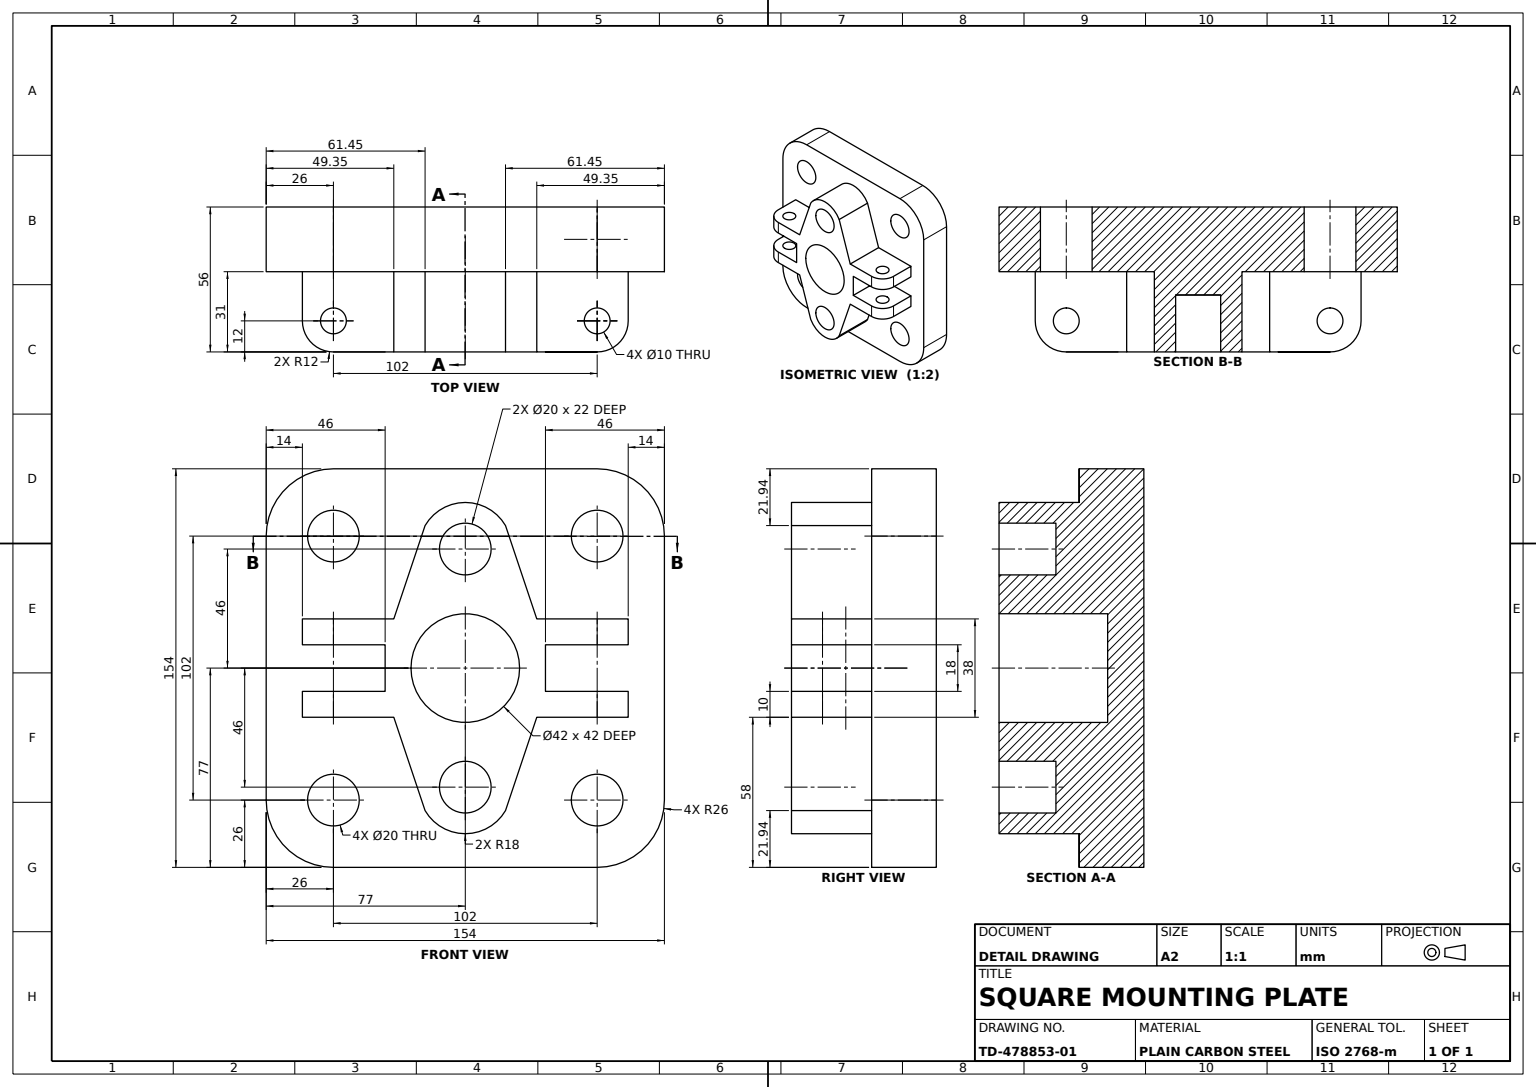
solid
v1 (26,-68,49)
v2 (26,-68,39)
e1 v1 v2 CIRCLE(AX(P(26,-68,44),D(0,-1,0),D(0,0,-1)),5)
v3 (26,-58,39)
e2 v3 v2 LINE
v4 (26,-58,49)
e3 v3 v4 CIRCLE(AX(P(26,-58,44),D(0,1,0),D(0,0,1)),5)
e4 v4 v1 LINE
face CYL(AX(P(26,-46,44),D(0,-1,0),D(0,0,-1)),5) rev [e1 -e2 e3 e4]
e5 v2 v1 CIRCLE(AX(P(26,-68,44),D(0,-1,0),D(0,0,-1)),5)
v5 (46,-68,56)
v6 (46,-68,25)
e6 v5 v6 LINE
v7 (26,-68,56)
e7 v5 v7 LINE
v8 (14,-68,44)
e8 v8 v7 CIRCLE(AX(P(26,-68,44),D(0,1,0),D(0,0,-1)),12)
v9 (14,-68,25)
e9 v8 v9 LINE
e10 v6 v9 LINE
face PLANE(AX(P(0,-68,56),D(0,-1,0),D(0,0,-1))) [-e5 -e1] [-e6 e7 -e8 e9 -e10]
v10 (128,-154,25)
v11 (128,-154,0)
e11 v10 v11 LINE
v12 (154,-128,0)
e12 v11 v12 CIRCLE(AX(P(128,-128,0),D(0,0,1),D(1,0,0)),26)
v13 (154,-128,25)
e13 v13 v12 LINE
e14 v10 v13 CIRCLE(AX(P(128,-128,25),D(0,0,1),D(1,0,0)),26)
face CYL(AX(P(128,-128,25),D(0,0,-1),D(-1,0,0)),26) [e11 e12 -e13 -e14]
v14 (154,-26,0)
e15 v12 v14 LINE
v15 (154,-26,25)
e16 v15 v14 LINE
e17 v13 v15 LINE
face PLANE(AX(P(154,-128,25),D(-1,0,0),D(0,0,1))) rev [e13 e15 -e16 -e17]
v16 (56,-77,14)
v17 (98,-77,14)
e18 v16 v17 CIRCLE(AX(P(77,-77,14),D(0,0,1),D(1,0,0)),21)
e19 v17 v16 CIRCLE(AX(P(77,-77,14),D(0,0,1),D(1,0,0)),21)
face PLANE(AX(P(77,-77,14),D(0,0,1),D(1,0,0))) [e18 e19]
v18 (36,-128,0)
v19 (16,-128,0)
e20 v18 v19 CIRCLE(AX(P(26,-128,0),D(0,0,1),D(1,0,0)),10)
v20 (36,-128,25)
e21 v18 v20 LINE
v21 (16,-128,25)
e22 v20 v21 CIRCLE(AX(P(26,-128,25),D(0,0,1),D(1,0,0)),10)
e23 v19 v21 LINE
face CYL(AX(P(26,-128,-17),D(0,0,1),D(1,0,0)),10) rev [-e20 e21 e22 -e23]
e24 v4 v3 CIRCLE(AX(P(26,-58,44),D(0,1,0),D(0,0,1)),5)
face CYL(AX(P(26,-46,44),D(0,-1,0),D(0,0,-1)),5) rev [e5 -e4 e24 e2]
v22 (67,-31,56)
v23 (87,-31,56)
e25 v22 v23 CIRCLE(AX(P(77,-31,56),D(0,0,1),D(1,0,0)),10)
e26 v23 v22 CIRCLE(AX(P(77,-31,56),D(0,0,1),D(1,0,0)),10)
v24 (87,-123,56)
v25 (67,-123,56)
e27 v24 v25 CIRCLE(AX(P(77,-123,56),D(0,0,1),D(1,0,0)),10)
e28 v25 v24 CIRCLE(AX(P(77,-123,56),D(0,0,1),D(1,0,0)),10)
v26 (92.552734,-21.938408,56)
v27 (61.447266,-21.938408,56)
e29 v26 v27 CIRCLE(AX(P(77,-31,56),D(0,0,1),D(1,0,0)),18)
v28 (49.353611,-58,56)
e30 v28 v27 LINE
v29 (26,-58,56)
e31 v29 v28 LINE
e32 v29 v7 LINE
v30 (46,-86,56)
e33 v30 v5 LINE
v31 (26,-86,56)
e34 v30 v31 LINE
v32 (26,-96,56)
e35 v31 v32 LINE
v33 (49.353611,-96,56)
e36 v32 v33 LINE
v34 (61.447266,-132.061592,56)
e37 v33 v34 LINE
v35 (92.552734,-132.061592,56)
e38 v34 v35 CIRCLE(AX(P(77,-123,56),D(0,0,1),D(1,0,0)),18)
v36 (104.646389,-96,56)
e39 v36 v35 LINE
v37 (128,-96,56)
e40 v37 v36 LINE
v38 (128,-86,56)
e41 v37 v38 LINE
v39 (108,-86,56)
e42 v39 v38 LINE
v40 (108,-68,56)
e43 v39 v40 LINE
v41 (128,-68,56)
e44 v40 v41 LINE
v42 (128,-58,56)
e45 v41 v42 LINE
v43 (104.646389,-58,56)
e46 v42 v43 LINE
e47 v43 v26 LINE
v44 (98,-77,56)
v45 (56,-77,56)
e48 v44 v45 CIRCLE(AX(P(77,-77,56),D(0,0,1),D(1,0,0)),21)
e49 v45 v44 CIRCLE(AX(P(77,-77,56),D(0,0,1),D(1,0,0)),21)
face PLANE(AX(P(0,0,56),D(0,0,1),D(1,0,0))) [-e25 -e26] [-e27 -e28] [e29 -e30 -e31 e32 -e7 -e33 e34 e35 e36 e37 e38 -e39 -e40 e41 -e42 e43 e44 e45 e46 e47] [-e48 -e49]
v46 (140,-96,44)
e50 v37 v46 CIRCLE(AX(P(128,-96,44),D(0,1,0),D(0,0,-1)),12)
v47 (140,-86,44)
e51 v47 v46 LINE
e52 v47 v38 CIRCLE(AX(P(128,-86,44),D(0,-1,0),D(0,0,1)),12)
face CYL(AX(P(128,-46,44),D(0,-1,0),D(0,0,-1)),12) [-e41 e50 -e51 e52]
v48 (26,-86,49)
v49 (26,-86,39)
e53 v48 v49 CIRCLE(AX(P(26,-86,44),D(0,-1,0),D(0,0,-1)),5)
e54 v49 v48 CIRCLE(AX(P(26,-86,44),D(0,-1,0),D(0,0,-1)),5)
v50 (46,-86,25)
v51 (14,-86,25)
e55 v50 v51 LINE
v52 (14,-86,44)
e56 v52 v51 LINE
e57 v52 v31 CIRCLE(AX(P(26,-86,44),D(0,1,0),D(0,0,-1)),12)
e58 v30 v50 LINE
face PLANE(AX(P(0,-86,56),D(0,-1,0),D(0,0,-1))) rev [e53 e54] [e55 -e56 e57 -e34 e58]
v53 (128,-86,49)
v54 (128,-86,39)
e59 v53 v54 CIRCLE(AX(P(128,-86,44),D(0,1,0),D(0,0,1)),5)
e60 v54 v53 CIRCLE(AX(P(128,-86,44),D(0,1,0),D(0,0,1)),5)
v55 (140,-86,25)
e61 v47 v55 LINE
v56 (108,-86,25)
e62 v56 v55 LINE
e63 v39 v56 LINE
face PLANE(AX(P(0,-86,56),D(0,1,0),D(0,0,1))) [-e59 -e60] [-e52 e61 -e62 -e63 e42]
v57 (14,-96,44)
v58 (14,-96,25)
e64 v57 v58 LINE
e65 v52 v57 LINE
e66 v51 v58 LINE
face PLANE(AX(P(14,0,56),D(1,0,0),D(0,0,-1))) rev [-e64 -e65 e56 e66]
v59 (138,-128,25)
v60 (118,-128,25)
e67 v59 v60 CIRCLE(AX(P(128,-128,25),D(0,0,1),D(1,0,0)),10)
v61 (118,-128,0)
e68 v61 v60 LINE
v62 (138,-128,0)
e69 v62 v61 CIRCLE(AX(P(128,-128,0),D(0,0,1),D(1,0,0)),10)
e70 v62 v59 LINE
face CYL(AX(P(128,-128,-17),D(0,0,1),D(1,0,0)),10) rev [e67 -e68 -e69 e70]
e71 v61 v62 CIRCLE(AX(P(128,-128,0),D(0,0,1),D(1,0,0)),10)
v63 (16,-26,0)
v64 (36,-26,0)
e72 v63 v64 CIRCLE(AX(P(26,-26,0),D(0,0,1),D(1,0,0)),10)
e73 v64 v63 CIRCLE(AX(P(26,-26,0),D(0,0,1),D(1,0,0)),10)
v65 (118,-26,0)
v66 (138,-26,0)
e74 v65 v66 CIRCLE(AX(P(128,-26,0),D(0,0,1),D(1,0,0)),10)
e75 v66 v65 CIRCLE(AX(P(128,-26,0),D(0,0,1),D(1,0,0)),10)
v67 (26,-154,0)
e76 v67 v11 LINE
v68 (0,-128,0)
e77 v68 v67 CIRCLE(AX(P(26,-128,0),D(0,0,1),D(1,0,0)),26)
v69 (0,-26,0)
e78 v69 v68 LINE
v70 (26,0,0)
e79 v70 v69 CIRCLE(AX(P(26,-26,0),D(0,0,1),D(1,0,0)),26)
v71 (128,0,0)
e80 v71 v70 LINE
e81 v14 v71 CIRCLE(AX(P(128,-26,0),D(0,0,1),D(-1,0,0)),26)
e82 v19 v18 CIRCLE(AX(P(26,-128,0),D(0,0,1),D(1,0,0)),10)
face PLANE(AX(P(26,-128,0),D(0,0,1),D(1,0,0))) rev [e71 e69] [e72 e73] [e74 e75] [-e15 -e12 -e76 -e77 -e78 -e79 -e80 -e81] [e82 e20]
v72 (128,-58,39)
v73 (128,-58,49)
e83 v72 v73 CIRCLE(AX(P(128,-58,44),D(0,-1,0),D(0,0,-1)),5)
v74 (128,-68,39)
e84 v72 v74 LINE
v75 (128,-68,49)
e85 v75 v74 CIRCLE(AX(P(128,-68,44),D(0,1,0),D(0,0,1)),5)
e86 v73 v75 LINE
face CYL(AX(P(128,-46,44),D(0,-1,0),D(0,0,-1)),5) rev [-e83 e84 -e85 -e86]
v76 (14,-58,25)
e87 v9 v76 LINE
v77 (14,-58,44)
e88 v77 v8 LINE
e89 v77 v76 LINE
face PLANE(AX(P(14,0,56),D(-1,0,0),D(0,0,1))) [-e87 -e9 -e88 e89]
e90 v74 v75 CIRCLE(AX(P(128,-68,44),D(0,1,0),D(0,0,1)),5)
e91 v73 v72 CIRCLE(AX(P(128,-58,44),D(0,-1,0),D(0,0,-1)),5)
face CYL(AX(P(128,-46,44),D(0,-1,0),D(0,0,-1)),5) rev [e86 -e90 -e84 -e91]
e92 v29 v77 CIRCLE(AX(P(26,-58,44),D(0,-1,0),D(0,0,1)),12)
face CYL(AX(P(26,-46,44),D(0,-1,0),D(0,0,-1)),12) [e88 e8 -e32 e92]
v78 (61.447266,-21.938408,25)
e93 v27 v78 LINE
v79 (92.552734,-21.938408,25)
e94 v26 v79 LINE
e95 v79 v78 CIRCLE(AX(P(77,-31,25),D(0,0,1),D(1,0,0)),18)
face CYL(AX(P(77,-31,56),D(0,0,-1),D(-1,0,0)),18) [-e93 -e29 e94 e95]
v80 (108,-68,25)
e96 v56 v80 LINE
e97 v40 v80 LINE
face PLANE(AX(P(108,0,56),D(-1,0,0),D(0,0,1))) rev [e96 -e97 -e43 e63]
e98 v60 v59 CIRCLE(AX(P(128,-128,25),D(0,0,1),D(1,0,0)),10)
face CYL(AX(P(128,-128,-17),D(0,0,1),D(1,0,0)),10) rev [-e71 e68 e98 -e70]
v81 (26,-96,49)
e99 v48 v81 LINE
v82 (26,-96,39)
e100 v81 v82 CIRCLE(AX(P(26,-96,44),D(0,-1,0),D(0,0,-1)),5)
e101 v49 v82 LINE
face CYL(AX(P(26,-46,44),D(0,-1,0),D(0,0,-1)),5) rev [e99 e100 -e101 -e53]
v83 (104.646389,-96,25)
e102 v36 v83 LINE
v84 (92.552734,-132.061592,25)
e103 v35 v84 LINE
e104 v83 v84 LINE
face PLANE(AX(P(123.006836,-41.251706,56),D(0.948104963,-0.317957511,0),D(0.317957511,0.948104963,0))) [-e102 e39 e103 -e104]
v85 (87,-31,34)
v86 (67,-31,34)
e105 v85 v86 CIRCLE(AX(P(77,-31,34),D(0,0,1),D(1,0,0)),10)
e106 v85 v23 LINE
e107 v86 v22 LINE
face CYL(AX(P(77,-31,34),D(0,0,1),D(1,0,0)),10) rev [-e105 e106 e26 -e107]
v87 (87,-123,34)
v88 (67,-123,34)
e108 v87 v88 CIRCLE(AX(P(77,-123,34),D(0,0,1),D(1,0,0)),10)
e109 v88 v87 CIRCLE(AX(P(77,-123,34),D(0,0,1),D(1,0,0)),10)
face PLANE(AX(P(77,-123,34),D(0,0,1),D(1,0,0))) [e108 e109]
e110 v82 v81 CIRCLE(AX(P(26,-96,44),D(0,-1,0),D(0,0,-1)),5)
face CYL(AX(P(26,-46,44),D(0,-1,0),D(0,0,-1)),5) rev [e101 e110 -e99 -e54]
e111 v17 v44 LINE
e112 v16 v45 LINE
face CYL(AX(P(77,-77,14),D(0,0,1),D(1,0,0)),21) rev [-e111 -e18 e112 e49]
e113 v50 v6 LINE
face PLANE(AX(P(46,0,56),D(-1,0,0),D(0,0,1))) [-e58 e33 e6 -e113]
v89 (140,-58,44)
v90 (140,-68,44)
e114 v89 v90 LINE
v91 (140,-68,25)
e115 v90 v91 LINE
v92 (140,-58,25)
e116 v91 v92 LINE
e117 v89 v92 LINE
face PLANE(AX(P(140,0,56),D(-1,0,0),D(0,0,1))) rev [e114 e115 e116 -e117]
v93 (49.353611,-96,25)
v94 (61.447266,-132.061592,25)
e118 v93 v94 LINE
e119 v34 v94 LINE
e120 v33 v93 LINE
face PLANE(AX(P(15.424229,5.172686,56),D(0.948104963,0.317957511,0),D(-0.317957511,0.948104963,0))) rev [e118 -e119 -e37 e120]
v95 (49.353611,-58,25)
e121 v95 v78 LINE
e122 v28 v95 LINE
face PLANE(AX(P(61.848621,-20.741621,56),D(-0.948104963,0.317957511,0),D(-0.317957511,-0.948104963,0))) [e30 e93 -e121 -e122]
e123 v58 v93 LINE
e124 v57 v32 CIRCLE(AX(P(26,-96,44),D(0,1,0),D(0,0,-1)),12)
face PLANE(AX(P(0,-96,56),D(0,1,0),D(0,0,1))) rev [-e100 -e110] [e123 -e120 -e36 -e124 e64]
v96 (128,-96,49)
v97 (128,-96,39)
e125 v96 v97 CIRCLE(AX(P(128,-96,44),D(0,-1,0),D(0,0,-1)),5)
e126 v54 v97 LINE
e127 v53 v96 LINE
face CYL(AX(P(128,-46,44),D(0,-1,0),D(0,0,-1)),5) rev [e125 -e126 e60 e127]
face CYL(AX(P(77,-77,14),D(0,0,1),D(1,0,0)),21) rev [e48 -e112 -e19 e111]
face CYL(AX(P(26,-46,44),D(0,-1,0),D(0,0,-1)),12) [-e57 e65 e124 -e35]
e128 v21 v20 CIRCLE(AX(P(26,-128,25),D(0,0,1),D(1,0,0)),10)
face CYL(AX(P(26,-128,-17),D(0,0,1),D(1,0,0)),10) rev [-e82 e23 e128 -e21]
v98 (104.646389,-58,25)
e129 v43 v98 LINE
e130 v98 v79 LINE
face PLANE(AX(P(76.582444,25.682772,56),D(-0.948104963,-0.317957511,0),D(0.317957511,-0.948104963,0))) rev [-e94 -e47 e129 e130]
e131 v88 v25 LINE
e132 v87 v24 LINE
face CYL(AX(P(77,-123,34),D(0,0,1),D(1,0,0)),10) rev [-e131 -e108 e132 e27]
e133 v97 v96 CIRCLE(AX(P(128,-96,44),D(0,-1,0),D(0,0,-1)),5)
v99 (140,-96,25)
e134 v46 v99 LINE
e135 v99 v83 LINE
face PLANE(AX(P(0,-96,56),D(0,-1,0),D(0,0,-1))) [-e133 -e125] [-e134 -e50 e40 e102 -e135]
e136 v86 v85 CIRCLE(AX(P(77,-31,34),D(0,0,1),D(1,0,0)),10)
face CYL(AX(P(77,-31,34),D(0,0,1),D(1,0,0)),10) rev [e25 -e106 -e136 e107]
v100 (118,-26,25)
v101 (138,-26,25)
e137 v100 v101 CIRCLE(AX(P(128,-26,25),D(0,0,1),D(1,0,0)),10)
e138 v66 v101 LINE
e139 v65 v100 LINE
face CYL(AX(P(128,-26,-17),D(0,0,1),D(1,0,0)),10) rev [e137 -e138 -e74 e139]
v102 (26,-154,25)
e140 v102 v67 LINE
v103 (0,-128,25)
e141 v103 v102 CIRCLE(AX(P(26,-128,25),D(0,0,1),D(1,0,0)),26)
e142 v103 v68 LINE
face CYL(AX(P(26,-128,25),D(0,0,-1),D(-1,0,0)),26) [-e140 -e141 e142 e77]
v104 (0,-26,25)
e143 v104 v69 LINE
v105 (26,0,25)
e144 v105 v104 CIRCLE(AX(P(26,-26,25),D(0,0,1),D(1,0,0)),26)
e145 v105 v70 LINE
face CYL(AX(P(26,-26,25),D(0,0,-1),D(-1,0,0)),26) [e79 -e143 -e144 e145]
v106 (128,0,25)
e146 v106 v105 LINE
e147 v106 v71 LINE
face PLANE(AX(P(128,0,25),D(0,-1,0),D(0,0,-1))) rev [-e146 e147 e80 -e145]
e148 v94 v84 CIRCLE(AX(P(77,-123,25),D(0,0,1),D(1,0,0)),18)
face CYL(AX(P(77,-123,56),D(0,0,-1),D(-1,0,0)),18) [-e38 e119 e148 -e103]
face PLANE(AX(P(77,-31,34),D(0,0,1),D(1,0,0))) [e136 e105]
e149 v80 v91 LINE
e150 v90 v41 CIRCLE(AX(P(128,-68,44),D(0,-1,0),D(0,0,1)),12)
face PLANE(AX(P(0,-68,56),D(0,1,0),D(0,0,1))) rev [-e44 e97 e149 -e115 e150] [e90 e85]
e151 v55 v99 LINE
face PLANE(AX(P(140,0,56),D(1,0,0),D(0,0,-1))) [-e151 -e61 e51 e134]
e152 v15 v106 CIRCLE(AX(P(128,-26,25),D(0,0,1),D(-1,0,0)),26)
face CYL(AX(P(128,-26,25),D(0,0,-1),D(-1,0,0)),26) [-e147 -e152 e16 e81]
e153 v102 v10 LINE
face PLANE(AX(P(26,-154,25),D(0,1,0),D(0,0,1))) rev [e140 e76 -e11 -e153]
e154 v76 v95 LINE
e155 v92 v98 LINE
v107 (36,-26,25)
v108 (16,-26,25)
e156 v107 v108 CIRCLE(AX(P(26,-26,25),D(0,0,1),D(1,0,0)),10)
e157 v108 v107 CIRCLE(AX(P(26,-26,25),D(0,0,1),D(1,0,0)),10)
e158 v104 v103 LINE
e159 v101 v100 CIRCLE(AX(P(128,-26,25),D(0,0,1),D(1,0,0)),10)
face PLANE(AX(P(26,-128,25),D(0,0,1),D(1,0,0))) [e10 e87 e154 e121 -e95 -e130 -e155 -e116 -e149 -e96 e62 e151 e135 e104 -e148 -e118 -e123 -e66 -e55 e113] [-e156 -e157] [-e98 -e67] [e152 e146 e144 e158 e141 e153 e14 e17] [-e159 -e137] [-e128 -e22]
face CYL(AX(P(77,-123,34),D(0,0,1),D(1,0,0)),10) rev [e28 -e132 -e109 e131]
e160 v63 v108 LINE
e161 v64 v107 LINE
face CYL(AX(P(26,-26,-17),D(0,0,1),D(1,0,0)),10) rev [e160 e157 -e161 -e72]
e162 v42 v89 CIRCLE(AX(P(128,-58,44),D(0,1,0),D(0,0,-1)),12)
face CYL(AX(P(128,-46,44),D(0,-1,0),D(0,0,-1)),12) [-e114 -e162 -e45 -e150]
face CYL(AX(P(128,-46,44),D(0,-1,0),D(0,0,-1)),5) rev [e59 e126 e133 -e127]
face PLANE(AX(P(0,-26,25),D(1,0,0),D(0,0,-1))) rev [-e142 -e158 e143 e78]
face PLANE(AX(P(0,-58,56),D(0,-1,0),D(0,0,-1))) rev [e91 e83] [e162 e117 e155 -e129 -e46]
face CYL(AX(P(26,-26,-17),D(0,0,1),D(1,0,0)),10) rev [-e73 e161 e156 -e160]
face PLANE(AX(P(0,-58,56),D(0,1,0),D(0,0,1))) [-e92 e31 e122 -e154 -e89] [-e24 -e3]
face CYL(AX(P(128,-26,-17),D(0,0,1),D(1,0,0)),10) rev [e159 -e139 -e75 e138]
